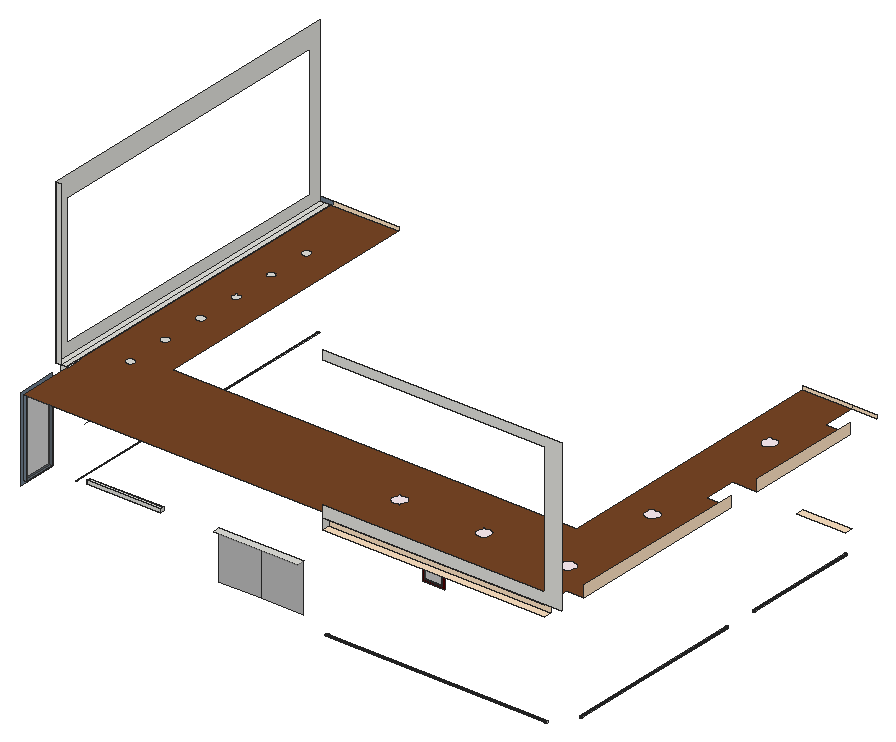
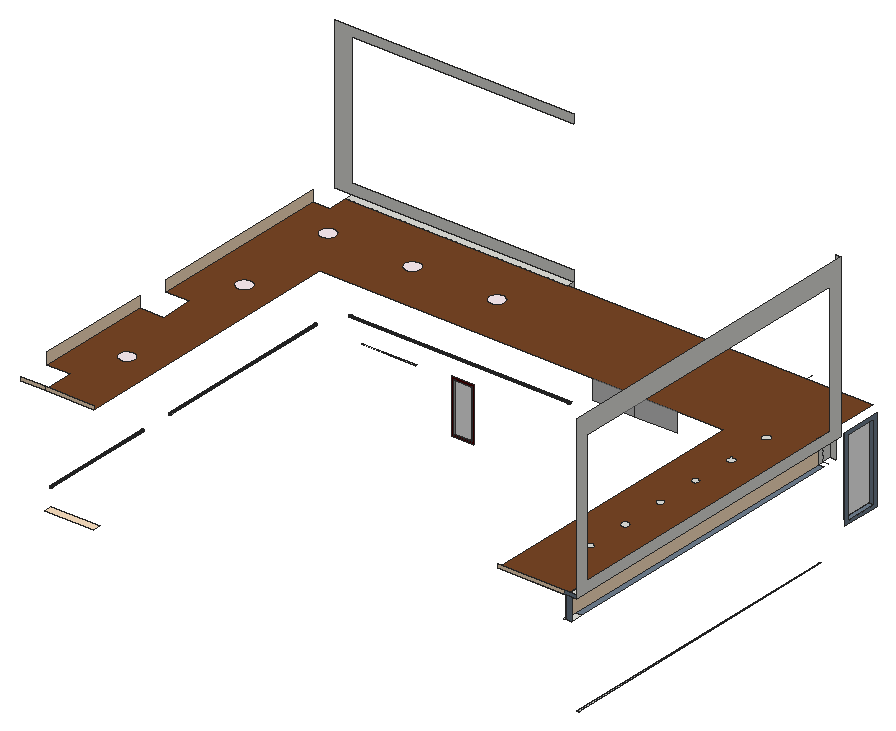
# SketchUp Ruby script. Lengths in inches.
U = 1.inch
M = Sketchup.active_model
def pt(a) = Geom::Point3d.new(a.map { |v| v * U })
def face(e, loops, mat)
  f = e.add_face(loops[0].map { |a| pt(a) })
  loops[1..].each { |l| e.add_face(l.map { |a| pt(a) }).erase! }
  f.material = f.back_material = mat if mat
  f
end
# faces: each face lists its corners as indices into pts; further lists are holes
def faces(e, pts, list, mat = nil) = list.each { |f| face(e, (f[0].is_a?(Array) ? f : [f]).map { |l| l.map { |i| pts[i] } }, mat) }
# xy, xz, yz: faces in a plane at the given z, y or x. An outline is a flat list of corners, or four numbers for a rectangle; further outlines are holes
def ring(l) = l.size == 4 ? [[l[0], l[1]], [l[2], l[1]], [l[2], l[3]], [l[0], l[3]]] : l.each_slice(2).to_a
def flat(e, list, mat, &to3) = list.each { |f| face(e, (f[0].is_a?(Array) ? f : [f]).map { |l| ring(l).map { |u, v| to3.(u, v) } }, mat) }
def xy(e, z, list, mat = nil) = flat(e, list, mat) { |x, y| [x, y, z] }
def xz(e, y, list, mat = nil) = flat(e, list, mat) { |x, z| [x, y, z] }
def yz(e, x, list, mat = nil) = flat(e, list, mat) { |y, z| [x, y, z] }
def lines(e, pts, list) = list.each { |a, b| e.add_line(pt(pts[a]), pt(pts[b])) }
# prism: a flat outline (further loops are holes) pulled along v
def prism(e, loops, v, mat = nil)
  f = face(e, loops, mat); d = Geom::Vector3d.new(v.map { |x| x * U })
  f.pushpull(f.normal.samedirection?(d) ? d.length : -d.length)
end
def box(e, o, s, mat = nil) = prism(e, [[o, [o[0] + s[0], o[1], o[2]], [o[0] + s[0], o[1] + s[1], o[2]], [o[0], o[1] + s[1], o[2]]]], [0, 0, s[2]], mat)
def at(x, y, z, deg = 0) = Geom::Transformation.translation(pt([x, y, z])) * Geom::Transformation.rotation(ORIGIN, Z_AXIS, deg.degrees)
def axes(o, x, y, z) = Geom::Transformation.new([*x, 0, *y, 0, *z, 0, *pt(o).to_a, 1])
def part(name) = M.definitions.add(name)
# library, detail: a bought-in or finely detailed component or shape, given as its bounding box
def library(name, o, s) = part(name).tap { |d| box(d.entities, o, s) }
def detail(e, o, s) = box(e.add_group.entities, o, s)
def put(e, d, t, mat = nil) = e.add_instance(d, t).tap { |i| i.material = mat if mat }
def group(e, t, mat = nil) = e.add_group.tap { |g| g.transformation = t; g.material = mat if mat }.entities
root = M.entities
M.materials.add("[0008_LavenderBlush]").color = [255, 240, 245]
M.materials.add("[0012_Bisque]").color = [255, 228, 196]
M.materials.add("[0021_DarkRed]").color = [76, 0, 0]
M.materials.add("[0111_SlateGray]").color = [112, 128, 144]
M.materials.add("[Translucent Glass Gray]").color = [84, 84, 84]
M.materials["[Translucent Glass Gray]"].alpha = 0.5
M.materials.add("[Translucent Resin Crush Gray]").color = [153, 153, 153]
M.materials["[Translucent Resin Crush Gray]"].alpha = 0.8
M.materials.add("[Wood Veneer 01]").color = [120, 70, 37]
box(root,[282.03,96,820.69],[240.38,12,10.38])
xy(root,627,[[1812,199.52,1813.5,798],[1812,906,1813.5,1284]])
xy(root,632.12,[[1584,1368,1745,1392]],"[0012_Bisque]")
xy(root,633,[[1044,118.5,1767.4375,120]])
xy(root,660.0625,[[1088.18,468,1145.12,469.5]])
xy(root,712.8125,[[24,158.55,36,264.68]],"[0111_SlateGray]")
xy(root,819.1875,[[1088.18,468,1145.12,469.5],[1268.41,468,1446.53,469.5]])
xy(root,825.43,[[695.08,96,971.45,120]])
xy(root,912,[[24,1350,42,1392],[42,1350,48,1392]])
xy(root,912,[[24,360,42,1350]],"[0111_SlateGray]")
xy(root,948,[[1044,108,1767.4375,132]],"[0012_Bisque]")
xy(root,962.8125,[[24,158.55,36,264.68]],"[0111_SlateGray]")
xy(root,984,[[1044,108,1767.4375,132],[6,312,24,1392],[24,312,42,1392],[42,312,48,342],[42,342,48,360],
  [151.96,423.39,148.86,423.84,145.98,425.07,143.52,427,141.64,429.51,140.47,432.41,140.1,435.52,140.54,438.625,141.77,441.51,143.7,443.97,146.21,445.85,149.12,447.02,152.23,447.39,155.33,446.95,158.21,445.72,160.67,443.78,162.55,441.28,163.72,438.37,164.1,435.26,163.65,432.16,162.42,429.28,160.49,426.8125,157.98,424.93,155.07,423.77],[151.96,567.39,148.86,567.84,145.98,569.07,143.52,571,141.64,573.51,140.47,576.41,140.1,579.52,140.54,582.625,141.77,585.51,143.7,587.97,146.21,589.85,149.12,591.02,152.23,591.39,155.33,590.95,158.21,589.72,160.67,587.78,162.55,585.28,163.72,582.37,164.1,579.26,163.65,576.16,162.42,573.28,160.49,570.8125,157.98,568.93,155.07,567.77],[151.96,711.39,148.86,711.84,145.98,713.07,143.52,715,141.64,717.51,140.47,720.41,140.1,723.52,140.54,726.625,141.77,729.51,143.7,731.97,146.21,733.85,149.12,735.02,152.23,735.39,155.33,734.95,158.21,733.72,160.67,731.78,162.55,729.28,163.72,726.37,164.1,723.26,163.65,720.16,162.42,717.28,160.49,714.8125,157.98,712.93,155.07,711.77],[151.96,855.39,148.86,855.84,145.98,857.07,143.52,859,141.64,861.51,140.47,864.41,140.1,867.52,140.54,870.625,141.77,873.51,143.7,875.97,146.21,877.85,149.12,879.02,152.23,879.39,155.33,878.95,158.21,877.72,160.67,875.78,162.55,873.28,163.72,870.37,164.1,867.26,163.65,864.16,162.42,861.28,160.49,858.8125,157.98,856.93,155.07,855.77],[151.96,999.39,148.86,999.84,145.98,1001.07,143.52,1003,141.64,1005.51,140.47,1008.41,140.1,1011.52,140.54,1014.625,141.77,1017.51,143.7,1019.97,146.21,1021.85,149.12,1023.02,152.23,1023.39,155.33,1022.95,158.21,1021.72,160.67,1019.78,162.55,1017.28,163.72,1014.37,164.1,1011.26,163.65,1008.16,162.42,1005.28,160.49,1002.8125,157.98,1000.93,155.07,999.77],
  [151.96,1143.39,148.86,1143.84,145.98,1145.07,143.52,1147,141.64,1149.51,140.47,1152.41,140.1,1155.52,140.54,1158.625,141.77,1161.51,143.7,1163.97,146.21,1165.85,149.12,1167.02,152.23,1167.39,155.33,1166.95,158.21,1165.72,160.67,1163.78,162.55,1161.28,163.72,1158.37,164.1,1155.26,163.65,1152.16,162.42,1149.28,160.49,1146.8125,157.98,1144.93,155.07,1143.77]])
xy(root,984,[[1135.91,278.18,1129.83,279.67,1124.34,282.69,1119.81,287.03,1116.57,292.39,1114.82,298.4,1114.69,304.67,1116.1875,310.75,1119.21,316.24,1123.54,320.76,1128.9,324.01,1134.92,325.76,1141.18,325.89,1147.27,324.39,1152.76,321.37,1157.28,317.04,1160.52,311.68,1162.27,305.66,1162.4,299.4,1160.91,293.3125,1157.89,287.82,1153.55,283.3,1148.19,280.06,1142.17,278.31],[1411.91,278.18,1405.83,279.67,1400.34,282.69,1395.81,287.03,1392.57,292.39,1390.82,298.4,1390.69,304.67,1392.1875,310.75,1395.21,316.24,1399.54,320.76,1404.9,324.01,1410.92,325.76,1417.18,325.89,1423.27,324.39,1428.76,321.37,1433.28,317.04,1436.52,311.68,1438.27,305.66,1438.4,299.4,1436.91,293.3125,1433.89,287.82,1429.55,283.3,1424.19,280.06,1418.17,278.31],[1687.91,278.18,1681.83,279.67,1676.34,282.69,1671.81,287.03,1668.57,292.39,1666.82,298.4,1666.69,304.67,1668.1875,310.75,1671.21,316.24,1675.54,320.76,1680.9,324.01,1686.92,325.76,1693.18,325.89,1699.27,324.39,1704.76,321.37,1709.28,317.04,1712.52,311.68,1714.27,305.66,1714.4,299.4,1712.91,293.3125,1709.89,287.82,1705.55,283.3,1700.19,280.06,1694.17,278.31],[1690.29,620.84,1684.08,621.65,1678.29,624.05,1673.32,627.87,1669.5,632.84,1667.11,638.625,1666.29,644.84,1667.11,651.05,1669.5,656.84,1673.32,661.81,1678.29,665.62,1684.08,668.02,1690.29,668.84,1696.5,668.02,1702.29,665.62,1707.26,661.81,1711.07,656.84,1713.47,651.05,1714.29,644.84,1713.47,638.625,1711.07,632.84,1707.26,627.87,1702.29,624.05,1696.5,621.65],[1690.29,1099.71,1684.08,1100.53,1678.29,1102.93,1673.32,1106.74,1669.5,1111.71,1667.11,1117.5,1666.29,1123.71,1667.11,1129.92,1669.5,1135.71,1673.32,1140.68,1678.29,1144.5,1684.08,1146.89,1690.29,1147.71,1696.5,1146.89,1702.29,1144.5,1707.26,1140.68,1711.07,1135.71,1713.47,1129.92,1714.29,1123.71,1713.47,1117.5,1711.07,1111.71,1707.26,1106.74,1702.29,1102.93,1696.5,1100.53]],"[0008_LavenderBlush]")
xy(root,984,[[[48,132,48,360,42,360,42,1392,264,1392,264,468,1584,468,1584,1392,1745,1392,1745,1284,1824,1284,1824,906,1745,906,1745,798,1824,798,1824,199.52,1767.4375,199.52,1767.4375,132],[1135.91,278.18,1142.17,278.31,1148.19,280.06,1153.55,283.3,1157.89,287.82,1160.91,293.3125,1162.4,299.4,1162.27,305.66,1160.52,311.68,1157.28,317.04,1152.76,321.37,1147.27,324.39,1141.18,325.89,1134.92,325.76,1128.9,324.01,1123.54,320.76,1119.21,316.24,1116.1875,310.75,1114.69,304.67,1114.82,298.4,1116.57,292.39,1119.81,287.03,1124.34,282.69,1129.83,279.67],[1687.91,278.18,1694.17,278.31,1700.19,280.06,1705.55,283.3,1709.89,287.82,1712.91,293.3125,1714.4,299.4,1714.27,305.66,1712.52,311.68,1709.28,317.04,1704.76,321.37,1699.27,324.39,1693.18,325.89,1686.92,325.76,1680.9,324.01,1675.54,320.76,1671.21,316.24,1668.1875,310.75,1666.69,304.67,1666.82,298.4,1668.57,292.39,1671.81,287.03,1676.34,282.69,1681.83,279.67],[1411.91,278.18,1418.17,278.31,1424.19,280.06,1429.55,283.3,1433.89,287.82,1436.91,293.3125,1438.4,299.4,1438.27,305.66,1436.52,311.68,1433.28,317.04,1428.76,321.37,1423.27,324.39,1417.18,325.89,1410.92,325.76,1404.9,324.01,1399.54,320.76,1395.21,316.24,1392.1875,310.75,1390.69,304.67,1390.82,298.4,1392.57,292.39,1395.81,287.03,1400.34,282.69,1405.83,279.67],[1690.29,620.84,1696.5,621.65,1702.29,624.05,1707.26,627.87,1711.07,632.84,1713.47,638.625,1714.29,644.84,1713.47,651.05,1711.07,656.84,1707.26,661.81,1702.29,665.62,1696.5,668.02,1690.29,668.84,1684.08,668.02,1678.29,665.62,1673.32,661.81,1669.5,656.84,1667.11,651.05,1666.29,644.84,1667.11,638.625,1669.5,632.84,1673.32,627.87,1678.29,624.05,1684.08,621.65],[1690.29,1099.71,1696.5,1100.53,1702.29,1102.93,1707.26,1106.74,1711.07,1111.71,1713.47,1117.5,1714.29,1123.71,1713.47,1129.92,1711.07,1135.71,1707.26,1140.68,1702.29,1144.5,1696.5,1146.89,1690.29,1147.71,1684.08,1146.89,1678.29,1144.5,1673.32,1140.68,1669.5,1135.71,1667.11,1129.92,1666.29,1123.71,1667.11,1117.5,1669.5,1111.71,1673.32,1106.74,1678.29,1102.93,1684.08,1100.53],[151.96,999.39,155.07,999.77,157.98,1000.93,160.49,1002.8125,162.42,1005.28,163.65,1008.16,164.1,1011.26,163.72,1014.37,162.55,1017.28,160.67,1019.78,158.21,1021.72,155.33,1022.95,152.23,1023.39,149.12,1023.02,146.21,1021.85,143.7,1019.97,141.77,1017.51,140.54,1014.625,140.1,1011.52,140.47,1008.41,141.64,1005.51,143.52,1003,145.98,1001.07,148.86,999.84],[151.96,855.39,155.07,855.77,157.98,856.93,160.49,858.8125,162.42,861.28,163.65,864.16,164.1,867.26,163.72,870.37,162.55,873.28,160.67,875.78,158.21,877.72,155.33,878.95,152.23,879.39,149.12,879.02,146.21,877.85,143.7,875.97,141.77,873.51,140.54,870.625,140.1,867.52,140.47,864.41,141.64,861.51,143.52,859,145.98,857.07,148.86,855.84],[151.96,711.39,155.07,711.77,157.98,712.93,160.49,714.8125,162.42,717.28,163.65,720.16,164.1,723.26,163.72,726.37,162.55,729.28,160.67,731.78,158.21,733.72,155.33,734.95,152.23,735.39,149.12,735.02,146.21,733.85,143.7,731.97,141.77,729.51,140.54,726.625,140.1,723.52,140.47,720.41,141.64,717.51,143.52,715,145.98,713.07,148.86,711.84],[151.96,567.39,155.07,567.77,157.98,568.93,160.49,570.8125,162.42,573.28,163.65,576.16,164.1,579.26,163.72,582.37,162.55,585.28,160.67,587.78,158.21,589.72,155.33,590.95,152.23,591.39,149.12,591.02,146.21,589.85,143.7,587.97,141.77,585.51,140.54,582.625,140.1,579.52,140.47,576.41,141.64,573.51,143.52,571,145.98,569.07,148.86,567.84],[151.96,423.39,155.07,423.77,157.98,424.93,160.49,426.8125,162.42,429.28,163.65,432.16,164.1,435.26,163.72,438.37,162.55,441.28,160.67,443.78,158.21,445.72,155.33,446.95,152.23,447.39,149.12,447.02,146.21,445.85,143.7,443.97,141.77,441.51,140.54,438.625,140.1,435.52,140.47,432.41,141.64,429.51,143.52,427,145.98,425.07,148.86,423.84],[151.96,1143.39,155.07,1143.77,157.98,1144.93,160.49,1146.8125,162.42,1149.28,163.65,1152.16,164.1,1155.26,163.72,1158.37,162.55,1161.28,160.67,1163.78,158.21,1165.72,155.33,1166.95,152.23,1167.39,149.12,1167.02,146.21,1165.85,143.7,1163.97,141.77,1161.51,140.54,1158.625,140.1,1155.52,140.47,1152.41,141.64,1149.51,143.52,1147,145.98,1145.07,148.86,1143.84]]],"[Wood Veneer 01]")
xz(root,108,[[1044,984,1824,984,1824,1476,1044,1476,1044,1446,1767.4375,1446,1767.4375,1020,1044,1020]])
xz(root,120,[[1044,633,1767.4375,636]])
xz(root,120,[[695.08,666.55,833.27,825.43],[833.27,666.55,971.45,825.43]],"[Translucent Resin Crush Gray]")
xz(root,132,[[1044,948,1767.4375,984]],"[0012_Bisque]")
xz(root,158.55,[[24,712.8125,36,962.8125]],"[0111_SlateGray]")
xz(root,199.52,[[1812,627,1812.78,627.1,1813.5,627.4,1814.12,627.88,1814.6,628.5,1814.9,629.22,1815,630,1814.9,630.78,1814.6,631.5,1814.12,632.12,1813.5,632.6,1812.78,632.9,1812,633,1811.22,632.9,1810.5,632.6,1809.88,632.12,1809.4,631.5,1809.1,630.78,1809,630,1809.1,629.22,1809.4,628.5,1809.88,627.88,1810.5,627.4,1811.22,627.1]])
xz(root,264.68,[[24,712.8125,36,962.8125]],"[0111_SlateGray]")
xz(root,312,[[24,912,42,984],[6,984,24,1512]])
xz(root,468,[[[1080.18,652.0625,1153.12,827.1875],[1088.18,660.0625,1145.12,819.1875]]],"[0021_DarkRed]")
xz(root,469.5,[[1088.18,660.0625,1145.12,819.1875]],"[Translucent Glass Gray]")
xz(root,1284,[[1812,627,1811.22,627.1,1810.5,627.4,1809.88,627.88,1809.4,628.5,1809.1,629.22,1809,630,1809.1,630.78,1809.4,631.5,1809.88,632.12,1810.5,632.6,1811.22,632.9,1812,633,1812.78,632.9,1813.5,632.6,1814.12,632.12,1814.6,631.5,1814.9,630.78,1815,630,1814.9,629.22,1814.6,628.5,1814.12,627.88,1813.5,627.4,1812.78,627.1]])
xz(root,1392,[[48,984,264,996],[1584,984,1745,996],[1745,984,1824,996]],"[0012_Bisque]")
xz(root,1392,[[24,912,42,984],[6,984,48,996]],"[0111_SlateGray]")
yz(root,6,[[[312,984,1392,1512],[360,1020,1350,1445.3125]]])
yz(root,24,[[[146.55,700.8125,276.68,974.8125],[158.55,712.8125,264.68,962.8125]]],"[0111_SlateGray]")
yz(root,36,[[158.55,712.8125,264.68,962.8125]],"[Translucent Glass Gray]")
yz(root,42,[[312,912,342,984],[342,912,360,984]])
yz(root,42,[[360,912,1392,984]],"[0012_Bisque]")
yz(root,1044,[[108,948,132,984]])
yz(root,1088.18,[[468,660.0625,469.5,819.1875]])
yz(root,1145.12,[[468,660.0625,469.5,819.1875]])
yz(root,1767.4375,[[120,633,120.78,633.1,121.5,633.4,122.12,633.88,122.6,634.5,122.9,635.22,123,636,122.9,636.78,122.6,637.5,122.12,638.12,121.5,638.6,120.78,638.9,120,639,119.22,638.9,118.5,638.6,117.88,638.12,117.4,637.5,117.1,636.78,117,636,117.1,635.22,117.4,634.5,117.88,633.88,118.5,633.4,119.22,633.1]])
yz(root,1812,[[199.52,627,798,630],[906,627,1284,630]])
yz(root,1824,[[199.52,984,798,1020],[906,984,1284,1020]],"[0012_Bisque]")
p = [[34.5,1350,626.6],[33.88,1350,626.12],[33.88,360,626.12],[34.5,360,626.6],[38.12,1350,626.12],[37.5,1350,626.6],
  [37.5,360,626.6],[38.12,360,626.12],[35.22,1350,626.9],[35.22,360,626.9],[36.78,1350,626.9],[36.78,360,626.9],
  [36,1350,627],[36,360,627],[1812,199.52,627],[1811.22,199.52,627.1],[1811.22,798,627.1],[1812,798,627],
  [1812.78,199.52,627.1],[1812.78,798,627.1],[1811.22,1284,627.1],[1812,1284,627],[1812,906,627],[1811.22,906,627.1],
  [1812.78,1284,627.1],[1812.78,906,627.1],[1810.5,199.52,627.4],[1810.5,798,627.4],[1813.5,199.52,627.4],[1813.5,798,627.4],
  [1810.5,1284,627.4],[1810.5,906,627.4],[1813.5,1284,627.4],[1813.5,906,627.4],[1809.88,199.52,627.88],[1809.88,798,627.88],
  [1814.12,199.52,627.88],[1814.12,798,627.88],[1809.88,1284,627.88],[1809.88,906,627.88],[1814.12,1284,627.88],[1814.12,906,627.88],
  [1809.4,199.52,628.5],[1809.4,798,628.5],[1814.6,199.52,628.5],[1814.6,798,628.5],[1809.4,1284,628.5],[1809.4,906,628.5],
  [1814.6,1284,628.5],[1814.6,906,628.5],[1809.1,199.52,629.22],[1809.1,798,629.22],[1814.9,199.52,629.22],[1814.9,798,629.22],
  [1809.1,1284,629.22],[1809.1,906,629.22],[1814.9,1284,629.22],[1814.9,906,629.22],[1809,199.52,630],[1809,798,630],
  [1815,199.52,630],[1815,798,630],[1809,1284,630],[1809,906,630],[1815,1284,630],[1815,906,630],
  [1809.1,199.52,630.78],[1809.1,798,630.78],[1814.9,199.52,630.78],[1814.9,798,630.78],[1809.1,1284,630.78],[1809.1,906,630.78],
  [1814.9,1284,630.78],[1814.9,906,630.78],[1809.4,199.52,631.5],[1809.4,798,631.5],[1814.6,199.52,631.5],[1814.6,798,631.5],
  [1809.4,1284,631.5],[1809.4,906,631.5],[1814.6,1284,631.5],[1814.6,906,631.5],[1809.88,199.52,632.12],[1809.88,798,632.12],
  [1814.12,199.52,632.12],[1814.12,798,632.12],[1809.88,1284,632.12],[1809.88,906,632.12],[1814.12,1284,632.12],[1814.12,906,632.12],
  [1810.5,199.52,632.6],[1810.5,798,632.6],[1813.5,199.52,632.6],[1813.5,798,632.6],[1810.5,1284,632.6],[1810.5,906,632.6],
  [1813.5,1284,632.6],[1813.5,906,632.6],[1811.22,199.52,632.9],[1811.22,798,632.9],[1812.78,199.52,632.9],[1812.78,798,632.9],
  [1811.22,1284,632.9],[1811.22,906,632.9],[1812.78,1284,632.9],[1812.78,906,632.9],[1812,199.52,633],[1812,798,633],
  [1812,1284,633],[1812,906,633],[1767.4375,120,633],[1767.4375,119.22,633.1],[1044,119.22,633.1],[1044,120,633],
  [1767.4375,120.78,633.1],[1044,120.78,633.1],[1767.4375,118.5,633.4],[1044,118.5,633.4],[1767.4375,121.5,633.4],[1044,121.5,633.4],
  [1767.4375,117.88,633.88],[1044,117.88,633.88],[1767.4375,122.12,633.88],[1044,122.12,633.88],[1767.4375,117.4,634.5],[1044,117.4,634.5],
  [1767.4375,122.6,634.5],[1044,122.6,634.5],[1767.4375,117.1,635.22],[1044,117.1,635.22],[1767.4375,122.9,635.22],[1044,122.9,635.22],
  [1767.4375,117,636],[1044,117,636],[1767.4375,123,636],[1044,123,636],[1767.4375,117.1,636.78],[1044,117.1,636.78],
  [1767.4375,122.9,636.78],[1044,122.9,636.78],[1767.4375,117.4,637.5],[1044,117.4,637.5],[1767.4375,122.6,637.5],[1044,122.6,637.5],
  [1767.4375,117.88,638.12],[1044,117.88,638.12],[1767.4375,122.12,638.12],[1044,122.12,638.12],[1767.4375,118.5,638.6],[1044,118.5,638.6],
  [1767.4375,121.5,638.6],[1044,121.5,638.6],[1767.4375,119.22,638.9],[1044,119.22,638.9],[1767.4375,120.78,638.9],[1044,120.78,638.9],
  [1767.4375,120,639],[1044,120,639],[264,132,984],[264,108,984],[42,342,912],[24,342,912]]
faces(root,p,[[0,1,2,3],[4,5,6,7],[8,0,3,9],[5,10,11,6],[12,8,9,13],[10,12,13,11],[14,15,16,17],[18,14,17,19],
  [20,21,22,23],[21,24,25,22],[15,26,27,16],[28,18,19,29],[30,20,23,31],[24,32,33,25],[26,34,35,27],[36,28,29,37],
  [38,30,31,39],[32,40,41,33],[34,42,43,35],[44,36,37,45],[46,38,39,47],[40,48,49,41],[42,50,51,43],[52,44,45,53],
  [54,46,47,55],[48,56,57,49],[50,58,59,51],[60,52,53,61],[62,54,55,63],[56,64,65,57],[58,66,67,59],[68,60,61,69],
  [70,62,63,71],[64,72,73,65],[66,74,75,67],[76,68,69,77],[78,70,71,79],[72,80,81,73],[74,82,83,75],[84,76,77,85],
  [86,78,79,87],[80,88,89,81],[82,90,91,83],[92,84,85,93],[94,86,87,95],[88,96,97,89],[90,98,99,91],[100,92,93,101],
  [102,94,95,103],[96,104,105,97],[98,106,107,99],[106,100,101,107],[108,102,103,109],[104,108,109,105],[110,111,112,113],[114,110,113,115],
  [111,116,117,112],[118,114,115,119],[116,120,121,117],[122,118,119,123],[120,124,125,121],[126,122,123,127],[124,128,129,125],[130,126,127,131],
  [128,132,133,129],[134,130,131,135],[132,136,137,133],[138,134,135,139],[136,140,141,137],[142,138,139,143],[140,144,145,141],[146,142,143,147],
  [144,148,149,145],[150,146,147,151],[148,152,153,149],[154,150,151,155],[152,156,157,153],[156,154,155,157]])
lines(root,p,[[158,159],[160,161]])
